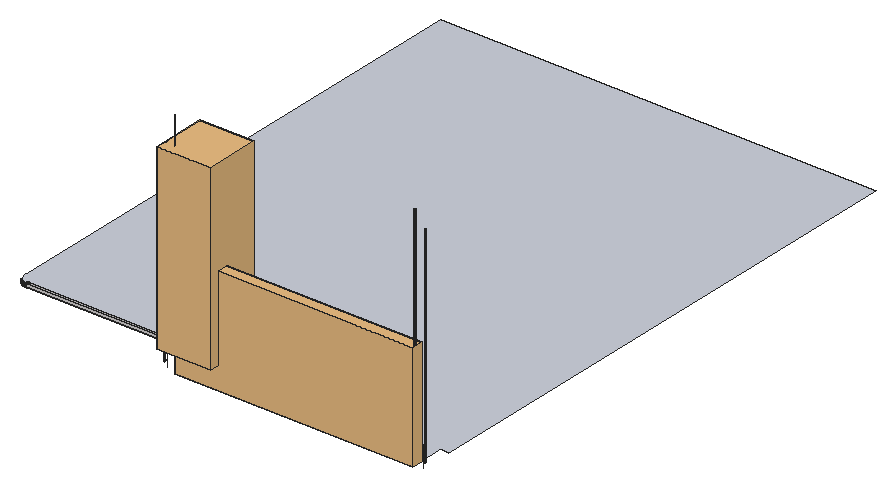
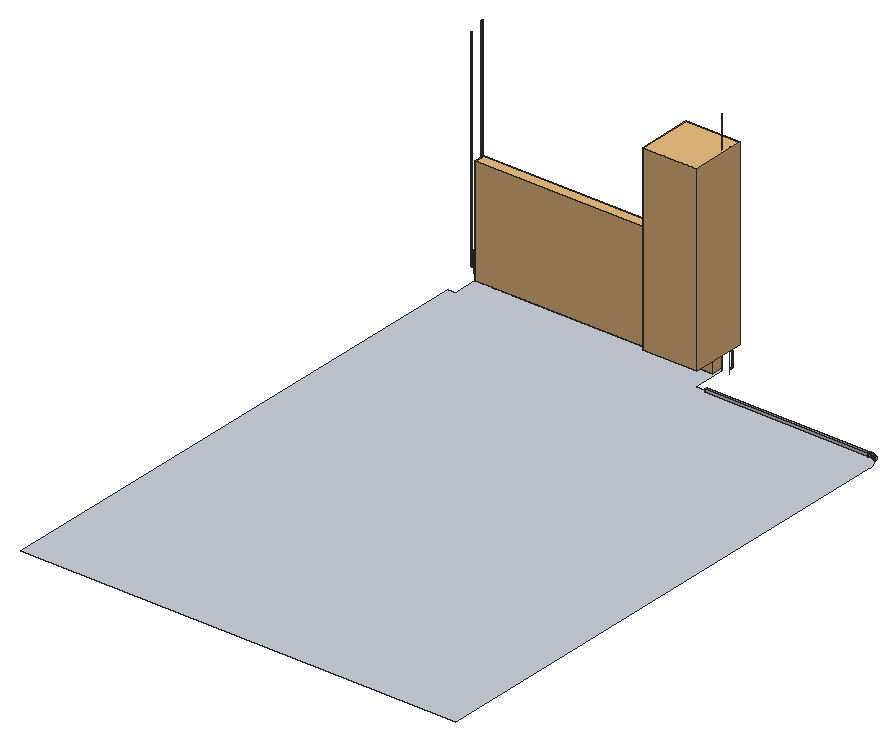
# SketchUp Ruby script. Lengths in inches.
U = 1.inch
M = Sketchup.active_model
def pt(a) = Geom::Point3d.new(a.map { |v| v * U })
def face(e, loops, mat)
  f = e.add_face(loops[0].map { |a| pt(a) })
  loops[1..].each { |l| e.add_face(l.map { |a| pt(a) }).erase! }
  f.material = f.back_material = mat if mat
  f
end
# faces: each face lists its corners as indices into pts; further lists are holes
def faces(e, pts, list, mat = nil) = list.each { |f| face(e, (f[0].is_a?(Array) ? f : [f]).map { |l| l.map { |i| pts[i] } }, mat) }
# xy, xz, yz: faces in a plane at the given z, y or x. An outline is a flat list of corners, or four numbers for a rectangle; further outlines are holes
def ring(l) = l.size == 4 ? [[l[0], l[1]], [l[2], l[1]], [l[2], l[3]], [l[0], l[3]]] : l.each_slice(2).to_a
def flat(e, list, mat, &to3) = list.each { |f| face(e, (f[0].is_a?(Array) ? f : [f]).map { |l| ring(l).map { |u, v| to3.(u, v) } }, mat) }
def xy(e, z, list, mat = nil) = flat(e, list, mat) { |x, y| [x, y, z] }
def xz(e, y, list, mat = nil) = flat(e, list, mat) { |x, z| [x, y, z] }
def yz(e, x, list, mat = nil) = flat(e, list, mat) { |y, z| [x, y, z] }
def lines(e, pts, list) = list.each { |a, b| e.add_line(pt(pts[a]), pt(pts[b])) }
# prism: a flat outline (further loops are holes) pulled along v
def prism(e, loops, v, mat = nil)
  f = face(e, loops, mat); d = Geom::Vector3d.new(v.map { |x| x * U })
  f.pushpull(f.normal.samedirection?(d) ? d.length : -d.length)
end
def box(e, o, s, mat = nil) = prism(e, [[o, [o[0] + s[0], o[1], o[2]], [o[0] + s[0], o[1] + s[1], o[2]], [o[0], o[1] + s[1], o[2]]]], [0, 0, s[2]], mat)
def at(x, y, z, deg = 0) = Geom::Transformation.translation(pt([x, y, z])) * Geom::Transformation.rotation(ORIGIN, Z_AXIS, deg.degrees)
def axes(o, x, y, z) = Geom::Transformation.new([*x, 0, *y, 0, *z, 0, *pt(o).to_a, 1])
def part(name) = M.definitions.add(name)
# library, detail: a bought-in or finely detailed component or shape, given as its bounding box
def library(name, o, s) = part(name).tap { |d| box(d.entities, o, s) }
def detail(e, o, s) = box(e.add_group.entities, o, s)
def put(e, d, t, mat = nil) = e.add_instance(d, t).tap { |i| i.material = mat if mat }
def group(e, t, mat = nil) = e.add_group.tap { |g| g.transformation = t; g.material = mat if mat }.entities
root = M.entities
M.materials.add("[Marble Carrara Floor Tile]").color = [204, 208, 219]
M.materials.add("[Quartz Light Brown]").color = [215, 212, 212]
M.materials.add("[Wood Cherry Original]").color = [152, 86, 42]
c1 = library("Garniza_zaclona",[1.52,0,0],[127.96,8.15,78.72])
c2 = library("Group\#4",[-1.08,-1,0],[60.58,61,204])
xy(root,126,[[216,155,480.079,155,480.192,155.005,480.306,155.015,480.419,155.028,480.531,155.046,480.643,155.069,480.754,155.095,480.863,155.126,480.972,155.161,481.079,155.2,481.184,155.243,481.288,155.29,481.39,155.341,481.49,155.395,481.588,155.454,481.683,155.516,481.776,155.582,481.867,155.651,481.955,155.723,482.04,155.799,482.122,155.878,482.201,155.96,482.276,156.045,482.349,156.133,482.418,156.224,482.484,156.317,482.546,156.412,482.604,156.51,482.659,156.61,482.71,156.712,482.757,156.815,482.8,156.921,482.838,157.028,482.873,157.136,482.904,157.246,482.93,157.357,482.953,157.469,482.971,157.581,482.984,157.694,482.994,157.808,482.999,157.921,483,194,492,194,492,794,3,794,3,212,3.001,211.804,3.005,211.607,3.012,211.411,3.021,211.215,3.032,211.019,3.046,210.823,3.063,210.627,3.082,210.432,3.104,210.237,3.128,210.042,3.155,209.848,3.185,209.653,3.217,209.46,3.251,209.266,3.288,209.074,3.328,208.881,3.37,208.69,3.414,208.498,3.462,208.308,3.511,208.118,3.563,207.928,3.618,207.74,3.675,207.552,3.734,207.365,3.796,207.178,3.86,206.993,3.927,206.808,3.996,206.624,4.068,206.442,4.142,206.26,4.218,206.079,4.297,205.899,4.378,205.72,4.461,205.542,4.547,205.366,4.635,205.19,4.725,205.016,4.818,204.843,4.913,204.671,5.01,204.5,5.109,204.331,5.21,204.163,5.314,203.996,5.42,203.83,5.528,203.666,5.638,203.504,5.75,203.343,5.865,203.183,5.981,203.025,6.1,202.869,6.22,202.714,6.343,202.56,6.467,202.408,6.594,202.258,6.722,202.11,6.853,201.963,6.985,201.818,7.119,201.675,7.255,201.533,7.393,201.393,7.533,201.255,7.675,201.119,7.818,200.985,7.963,200.853,8.11,200.722,8.258,200.594,8.408,200.467,8.56,200.343,8.714,200.22,8.869,200.1,9.025,199.981,9.183,199.865,9.343,199.75,9.504,199.638,9.666,199.528,9.83,199.42,9.996,199.314,10.163,199.21,10.331,199.109,10.5,199.01,10.671,198.913,10.843,198.818,11.016,198.725,11.19,198.635,11.366,198.547,11.542,198.461,11.72,198.378,11.899,198.297,12.079,198.218,12.26,198.142,12.442,198.068,12.624,197.996,12.808,197.927,12.993,197.86,13.178,197.796,13.365,197.734,13.552,197.675,13.74,197.618,13.928,197.563,14.118,197.511,14.308,197.462,14.498,197.414,14.69,197.37,14.881,197.328,15.074,197.288,15.266,197.251,15.46,197.217,15.653,197.185,15.848,197.155,16.042,197.128,16.237,197.104,16.432,197.082,16.627,197.063,16.823,197.046,17.019,197.032,17.215,197.021,17.411,197.012,17.607,197.005,17.804,197.001,18,197,201,197,201,194,213,194,213,158,213.002,157.882,213.009,157.765,213.021,157.647,213.037,157.531,213.058,157.415,213.083,157.3,213.113,157.186,213.147,157.073,213.186,156.962,213.229,156.852,213.276,156.744,213.327,156.638,213.383,156.534,213.442,156.433,213.506,156.333,213.573,156.237,213.644,156.143,213.719,156.052,213.797,155.964,213.879,155.879,213.964,155.797,214.052,155.719,214.143,155.644,214.237,155.573,214.333,155.506,214.433,155.442,214.534,155.383,214.638,155.327,214.744,155.276,214.852,155.228,214.962,155.185,215.073,155.147,215.186,155.113,215.3,155.083,215.415,155.058,215.531,155.037,215.648,155.021,215.765,155.009,215.882,155.002]],"[Marble Carrara Floor Tile]")
xz(root,194,[[18,126,201,129]],"[Quartz Light Brown]")
xz(root,194.5,[[18.002,125,201,126]],"[Quartz Light Brown]")
xz(root,197,[[18,126,201,129]],"[Quartz Light Brown]")
yz(root,201,[[194,125,194.5,126],[194,126,197,129]],"[Quartz Light Brown]")
yz(root,482.996,[[157.843,126,157.846,384]],"[Quartz Light Brown]")
p = [[16.627,194.554,126],[16.627,194.554,125],[16.855,194.537,125],[16.855,194.537,126],[17.084,194.524,125],[17.084,194.524,126],
  [17.313,194.514,125],[17.313,194.514,126],[17.542,194.506,125],[17.542,194.506,126],[17.771,194.502,125],[17.771,194.502,126],
  [18.002,194.5,125],[18.002,194.5,126],[15.489,194.681,126],[15.489,194.681,125],[15.716,194.65,125],[15.716,194.65,126],
  [15.943,194.621,125],[15.943,194.621,126],[16.171,194.596,125],[16.171,194.596,126],[16.399,194.573,125],[16.399,194.573,126],
  [15.036,194.753,126],[15.036,194.753,125],[15.262,194.715,125],[15.262,194.715,126],[14.362,194.882,126],[14.362,194.882,125],
  [14.586,194.836,125],[14.586,194.836,126],[14.811,194.793,125],[14.811,194.793,126],[13.915,194.984,126],[13.915,194.984,125],
  [14.138,194.932,125],[14.138,194.932,126],[13.471,195.096,126],[13.471,195.096,125],[13.692,195.038,125],[13.692,195.038,126],
  [13.25,195.157,126],[13.25,195.157,125],[12.811,195.287,126],[12.811,195.287,125],[13.03,195.221,125],[13.03,195.221,126],
  [12.592,195.357,126],[12.592,195.357,125],[12.158,195.504,126],[12.158,195.504,125],[12.375,195.429,125],[12.375,195.429,126],
  [11.943,195.582,126],[11.943,195.582,125],[11.729,195.662,126],[11.729,195.662,125],[11.303,195.832,126],[11.303,195.832,125],
  [11.515,195.746,125],[11.515,195.746,126],[11.092,195.921,126],[11.092,195.921,125],[10.882,196.013,126],[10.882,196.013,125],
  [10.673,196.108,126],[10.673,196.108,125],[10.466,196.205,126],[10.466,196.205,125],[10.26,196.305,126],[10.26,196.305,125],
  [10.055,196.407,126],[10.055,196.407,125],[9.852,196.513,126],[9.852,196.513,125],[9.65,196.621,126],[9.65,196.621,125],
  [9.449,196.731,126],[9.449,196.731,125],[9.25,196.845,126],[9.25,196.845,125],[9.052,196.96,126],[9.052,196.96,125],
  [8.856,197.079,126],[8.856,197.079,125],[8.662,197.2,126],[8.662,197.2,125],[8.469,197.323,126],[8.469,197.323,125],
  [8.278,197.449,126],[8.278,197.449,125],[213.506,156.333,384],[213.528,156.301,384],[213.528,156.301,126],[213.506,156.333,126],
  [213.484,156.366,384],[213.484,156.366,126],[482.494,156.333,384],[482.498,156.338,384],[482.498,156.338,126],[482.494,156.333,126],
  [482.516,156.366,126],[482.516,156.366,384],[213.442,156.433,384],[213.463,156.399,384],[213.463,156.399,126],[213.442,156.433,126],
  [213.422,156.466,384],[213.422,156.466,126],[482.537,156.399,384],[482.537,156.399,126],[482.541,156.405,384],[482.558,156.433,384],
  [482.558,156.433,126],[482.56,156.435,384],[482.56,156.435,126],[482.578,156.466,126],[482.576,156.462,384],[482.578,156.466,384],
  [213.402,156.5,384],[213.402,156.5,126],[213.383,156.534,384],[213.383,156.534,126],[213.364,156.569,384],[213.364,156.569,126],
  [482.598,156.5,384],[482.598,156.5,126],[482.602,156.507,384],[482.617,156.534,384],[482.617,156.534,126],[482.632,156.561,384],
  [482.636,156.569,384],[482.636,156.569,126],[213.345,156.603,384],[213.345,156.603,126],[213.327,156.638,384],[213.327,156.638,126],
  [213.309,156.673,384],[213.309,156.673,126],[482.655,156.603,384],[482.655,156.603,126],[482.659,156.61,384],[482.672,156.635,384],
  [482.672,156.635,126],[482.673,156.638,126],[482.673,156.638,384],[482.684,156.661,384],[482.691,156.673,384],[482.691,156.673,126],
  [213.292,156.708,384],[213.292,156.708,126],[213.276,156.744,384],[213.276,156.744,126],[213.259,156.78,384],[213.259,156.78,126],
  [482.708,156.708,384],[482.708,156.708,126],[482.711,156.716,384],[482.722,156.738,384],[482.722,156.738,126],[482.724,156.744,126],
  [482.724,156.744,384],[482.732,156.762,384],[482.741,156.78,384],[482.741,156.78,126],[213.244,156.816,384],[213.244,156.816,126],
  [213.228,156.852,384],[213.228,156.852,126],[482.756,156.816,384],[482.756,156.816,126],[482.76,156.823,384],[482.768,156.843,384],
  [482.768,156.843,126],[482.772,156.852,126],[482.772,156.852,384],[213.214,156.888,384],[213.214,156.888,126],[213.199,156.925,384],
  [213.199,156.925,126],[213.185,156.962,384],[213.185,156.962,126],[482.777,156.864,384],[482.786,156.888,384],[482.786,156.888,126],
  [482.801,156.925,384],[482.801,156.925,126],[482.804,156.932,384],[482.811,156.95,384],[482.81,156.95,126],[213.147,157.073,384],
  [213.159,157.036,384],[213.159,157.036,126],[213.147,157.073,126],[213.172,156.999,384],[213.172,156.999,126],[482.815,156.962,126],
  [482.815,156.962,384],[482.816,156.967,384],[482.828,156.999,384],[482.828,156.999,126],[482.841,157.036,384],[482.841,157.036,126],
  [482.843,157.043,384],[482.849,157.058,384],[482.849,157.058,126],[213.135,157.11,384],[213.135,157.11,126],[213.124,157.148,384],
  [213.124,157.148,126],[213.113,157.186,384],[213.113,157.186,126],[482.853,157.073,126],[482.853,157.071,384],[482.853,157.073,384],
  [482.865,157.11,384],[482.865,157.11,126],[482.876,157.148,384],[482.876,157.148,126],[482.878,157.155,384],[482.883,157.168,384],
  [482.882,157.168,126],[213.102,157.224,384],[213.102,157.224,126],[213.092,157.262,384],[213.092,157.262,126],[482.887,157.186,126],
  [482.886,157.18,384],[482.887,157.186,384],[482.898,157.224,384],[482.898,157.224,126],[482.908,157.262,384],[482.908,157.262,126],
  [213.083,157.3,384],[213.083,157.3,126],[213.074,157.338,384],[213.074,157.338,126],[213.066,157.376,384],[213.066,157.376,126],
  [482.909,157.268,384],[482.912,157.279,384],[482.912,157.279,126],[482.917,157.3,126],[482.915,157.29,384],[482.917,157.3,384],
  [482.926,157.338,384],[482.926,157.338,126],[482.934,157.376,384],[482.934,157.376,126],[213.058,157.415,384],[213.058,157.415,126],
  [213.05,157.453,384],[213.05,157.453,126],[482.936,157.382,384],[482.9375,157.391,384],[482.9375,157.391,126],[482.942,157.415,126],
  [482.94,157.401,384],[482.942,157.415,384],[482.95,157.453,384],[482.95,157.453,126],[213.043,157.492,384],[213.043,157.492,126],
  [213.037,157.531,384],[213.037,157.531,126],[213.031,157.57,384],[213.031,157.57,126],[482.957,157.492,384],[482.957,157.492,126],
  [482.958,157.497,384],[482.959,157.504,384],[482.959,157.504,126],[482.963,157.531,126],[482.96,157.512,384],[482.963,157.531,384],
  [482.969,157.57,384],[482.969,157.57,126],[213.026,157.608,384],[213.026,157.608,126],[213.021,157.647,384],[213.021,157.647,126],
  [213.016,157.686,384],[213.016,157.686,126],[482.974,157.608,384],[482.974,157.608,126],[482.975,157.613,384],[482.976,157.617,384],
  [482.976,157.617,126],[482.979,157.647,126],[482.976,157.623,384],[482.979,157.647,384],[482.984,157.686,384],[482.984,157.686,126],
  [213.013,157.725,384],[213.013,157.725,126],[213.009,157.765,384],[213.009,157.765,126],[482.987,157.725,384],[482.987,157.725,126],
  [482.988,157.729,384],[482.988,157.731,384],[482.988,157.731,126],[482.991,157.765,126],[482.988,157.735,384],[482.991,157.765,384],
  [213.006,157.804,384],[213.006,157.804,126],[213.004,157.843,384],[213.004,157.843,126],[213.002,157.881,126],[213.003,157.881,384],
  [482.994,157.804,384],[482.994,157.804,126],[482.996,157.843,384],[482.996,157.843,126],[482.998,157.882,126],[482.996,157.846,126],
  [482.996,157.846,384],[482.998,157.882,384],[213.002,157.882,384],[213.002,157.882,126],[213.001,157.921,384],[213.001,157.921,126],
  [482.999,157.921,384],[482.999,157.921,126],[16.823,194.039,126],[16.823,194.039,129],[16.588,194.055,129],[16.588,194.055,126],
  [17.058,194.025,126],[17.058,194.025,129],[17.293,194.014,126],[17.293,194.014,129],[17.529,194.006,126],[17.529,194.006,129],
  [17.764,194.002,126],[17.764,194.002,129],[18,194,126],[18,194,129],[15.884,194.125,126],[15.884,194.125,129],
  [15.651,194.154,129],[15.651,194.154,126],[16.118,194.099,126],[16.118,194.099,129],[16.353,194.076,126],[16.353,194.076,129],
  [15.184,194.222,126],[15.184,194.222,129],[14.952,194.26,129],[14.952,194.26,126],[15.417,194.186,126],[15.417,194.186,129],
  [14.488,194.346,126],[14.488,194.346,129],[14.258,194.393,129],[14.258,194.393,126],[14.72,194.301,126],[14.72,194.301,129],
  [14.027,194.444,126],[14.027,194.444,129],[13.798,194.497,129],[13.798,194.497,126],[13.569,194.554,129],[13.569,194.554,126],
  [13.341,194.613,126],[13.341,194.613,129],[13.114,194.676,129],[13.114,194.676,126],[12.888,194.741,126],[12.888,194.741,129],
  [12.662,194.81,129],[12.662,194.81,126],[12.4375,194.881,129],[12.4375,194.881,126],[12.214,194.955,129],[12.214,194.955,126],
  [11.991,195.032,126],[11.991,195.032,129],[11.77,195.113,129],[11.77,195.113,126],[11.549,195.196,129],[11.549,195.196,126],
  [11.33,195.281,129],[11.33,195.281,126],[11.112,195.37,129],[11.112,195.37,126],[10.895,195.462,129],[10.895,195.462,126],
  [10.679,195.556,129],[10.679,195.556,126],[10.464,195.653,129],[10.464,195.653,126],[10.251,195.753,129],[10.251,195.753,126],
  [10.039,195.856,129],[10.039,195.856,126],[9.828,195.962,129],[9.828,195.962,126],[9.619,196.07,129],[9.619,196.07,126],
  [9.411,196.181,129],[9.411,196.181,126],[9.205,196.295,129],[9.205,196.295,126],[9,196.412,129],[9,196.412,126],
  [8.797,196.531,129],[8.797,196.531,126],[8.595,196.652,129],[8.595,196.652,126],[8.395,196.777,129],[8.395,196.777,126],
  [8.196,196.904,129],[8.196,196.904,126],[8,197.034,129],[8,197.034,126],[7.805,197.166,129],[7.805,197.166,126],
  [16.823,197.046,126],[16.627,197.063,126],[16.627,197.063,129],[16.823,197.046,129],[17.019,197.032,126],[17.019,197.032,129],
  [17.215,197.021,126],[17.215,197.021,129],[17.411,197.012,126],[17.411,197.012,129],[17.607,197.005,126],[17.607,197.005,129],
  [17.804,197.001,126],[17.804,197.001,129],[18,197,126],[18,197,129],[16.042,197.128,126],[15.848,197.155,126],
  [15.848,197.155,129],[16.042,197.128,129],[16.237,197.104,126],[16.237,197.104,129],[16.432,197.082,126],[16.432,197.082,129],
  [7.611,197.3,129],[7.611,197.3,126],[15.46,197.217,126],[15.266,197.251,126],[15.266,197.251,129],[15.46,197.217,129],
  [15.653,197.185,126],[15.653,197.185,129],[7.42,197.4375,129],[7.42,197.4375,126],[14.881,197.328,126],[14.69,197.37,126],
  [14.69,197.37,129],[14.881,197.328,129],[15.074,197.288,126],[15.074,197.288,129],[202.077,156.537,133],[202.077,156.537,132],
  [202.097,156.354,132],[202.097,156.354,133],[493.903,156.354,133],[493.903,156.354,132],[493.923,156.537,132],[493.923,156.537,133],
  [202.059,156.719,133],[202.059,156.719,132],[493.941,156.719,132],[493.941,156.719,133],[202.043,156.902,133],[202.043,156.902,132],
  [493.957,156.902,132],[493.957,156.902,133],[202.03,157.084,133],[202.03,157.084,132],[493.97,157.084,132],[493.97,157.084,133],
  [202.019,157.267,133],[202.019,157.267,132],[493.981,157.267,132],[493.981,157.267,133],[202.011,157.45,133],[202.011,157.45,132],
  [493.989,157.45,132],[493.989,157.45,133],[202.005,157.634,133],[202.005,157.634,132],[493.995,157.634,132],[493.995,157.634,133],
  [202.001,157.817,133],[202.001,157.817,132],[493.999,157.817,132],[493.999,157.817,133],[202,158.003,133],[202,158.003,132],
  [494,158.003,132],[494,158.003,133],[201.104,156.237,133],[201.104,156.237,150],[201.082,156.432,150],[201.082,156.432,133],
  [494.896,156.237,368],[494.896,156.237,133],[494.918,156.432,133],[494.918,156.432,368],[201.063,156.627,150],[201.063,156.627,133],
  [494.937,156.627,133],[494.937,156.627,368],[201.046,156.823,150],[201.046,156.823,133],[494.954,156.823,133],[494.954,156.823,368],
  [201.032,157.019,150],[201.032,157.019,133],[494.968,157.019,133],[494.968,157.019,368],[201.021,157.215,150],[201.021,157.215,133],
  [494.979,157.215,133],[494.979,157.215,368],[201.012,157.411,150],[201.012,157.411,133],[494.988,157.411,133],[494.988,157.411,368],
  [201.005,157.607,150],[201.005,157.607,133],[494.995,157.607,133],[494.995,157.607,368],[201.001,157.804,150],[201.001,157.804,133],
  [494.999,157.804,133],[494.999,157.804,368],[201,158,150],[201,158,133],[495,158,133],[495,158,368],
  [201.828,156.51,150],[201.849,156.325,150],[201.849,156.325,149.75],[201.828,156.51,149.75],[202.345,156.384,150],[202.325,156.563,150],
  [202.325,156.563,149.75],[202.345,156.384,149.75],[201.81,156.696,150],[201.81,156.696,149.75],[202.308,156.742,150],[202.308,156.742,149.75],
  [201.794,156.882,150],[201.794,156.882,149.75],[202.292,156.921,150],[202.292,156.921,149.75],[201.781,157.068,150],[201.781,157.068,149.75],
  [202.279,157.101,150],[202.279,157.101,149.75],[201.77,157.254,150],[201.77,157.254,149.75],[202.269,157.28,150],[202.269,157.28,149.75],
  [201.761,157.441,150],[201.761,157.441,149.75],[202.261,157.46,150],[202.261,157.46,149.75],[201.755,157.627,150],[201.755,157.627,149.75],
  [202.255,157.64,150],[202.255,157.64,149.75],[201.751,157.813,150],[201.751,157.813,149.75],[202.251,157.82,150],[202.251,157.82,149.75],
  [201.75,158,150],[201.75,158,149.75],[202.25,158,150],[202.25,158,149.75],[204.124,156.278,150],[204.124,156.278,354],
  [204.103,156.434,354],[204.103,156.434,150],[204.083,156.59,354],[204.083,156.59,150],[204.066,156.746,354],[204.066,156.746,150],
  [204.05,156.902,354],[204.05,156.902,150],[204.037,157.058,354],[204.037,157.058,150],[204.026,157.215,354],[204.026,157.215,150],
  [204.016,157.372,354],[204.016,157.372,150],[204.009,157.529,354],[204.009,157.529,150],[204.004,157.686,354],[204.004,157.686,150],
  [204.001,157.843,354],[204.001,157.843,150],[204,158,354],[204,158,150],[492,158,150],[492,158,126],
  [204,158,126],[491.876,156.278,150],[491.897,156.434,150],[491.917,156.59,150],[491.934,156.746,150],[491.95,156.902,150],
  [491.963,157.058,150],[491.974,157.215,150],[491.984,157.372,150],[491.991,157.529,150],[491.996,157.686,150],[491.999,157.843,150]]
faces(root,p,[[0,1,2,3],[3,2,4,5],[5,4,6,7],[7,6,8,9],[9,8,10,11],[11,10,12,13],[14,15,16,17],[17,16,18,19],
  [19,18,20,21],[21,20,22,23],[23,22,1,0],[24,25,26,27],[27,26,15,14],[28,29,30,31],[31,30,32,33],[33,32,25,24],
  [34,35,36,37],[37,36,29,28],[38,39,40,41],[41,40,35,34],[42,43,39,38],[44,45,46,47],[47,46,43,42],[48,49,45,44],
  [50,51,52,53],[53,52,49,48],[54,55,51,50],[56,57,55,54],[58,59,60,61],[61,60,57,56],[62,63,59,58],[64,65,63,62],
  [66,67,65,64],[68,69,67,66],[70,71,69,68],[72,73,71,70],[74,75,73,72],[76,77,75,74],[78,79,77,76],[80,81,79,78],
  [82,83,81,80],[84,85,83,82],[86,87,85,84],[88,89,87,86],[90,91,89,88],[92,93,94,95],[96,92,95,97],[98,99,100,101],
  [102,100,99,103],[104,105,106,107],[108,104,107,109],[105,96,97,106],[103,110,111,102],[110,112,113,114,111],[113,115,116,114],[117,116,115,118,119],
  [120,108,109,121],[122,120,121,123],[124,122,123,125],[119,126,127,117],[126,128,129,130,127],[129,131,132,133,130],[134,124,125,135],[136,134,135,137],
  [138,136,137,139],[132,140,141,133],[142,143,144,141,140],[145,144,143,146],[146,147,148,149,145],[150,138,139,151],[152,150,151,153],[154,152,153,155],
  [148,156,157,149],[158,159,160,157,156],[161,160,159,162],[162,163,164,165,161],[166,154,155,167],[168,166,167,169],[164,170,171,165],[172,173,174,171,170],
  [175,174,173,176],[177,168,169,178],[179,177,178,180],[181,179,180,182],[176,183,184,185,175],[184,186,187,185],[188,189,190,187,186],[191,192,193,194],
  [195,181,182,196],[195,192,193,196],[197,190,189,198],[198,199,200,201,197],[200,202,203,201],[204,205,206,203,202],[207,191,194,208],[207,209,210,208],
  [211,209,210,212],[213,206,205,214,215],[215,216,217,213],[216,218,219,217],[220,221,222,219,218],[223,211,212,224],[225,223,224,226],[227,222,221,228,229],
  [229,230,231,227],[230,232,233,231],[234,225,226,235],[236,234,235,237],[238,236,237,239],[240,241,242,233,232],[243,242,241,244,245],[245,246,247,243],
  [246,248,249,247],[250,238,239,251],[252,250,251,253],[254,255,256,249,248],[257,256,255,258,259],[259,260,261,257],[262,252,253,263],[264,262,263,265],
  [266,264,265,267],[260,268,269,261],[270,271,272,269,268],[273,272,271,274,275],[275,276,277,273],[278,266,267,279],[280,278,279,281],[282,280,281,283],
  [276,284,285,277],[286,287,288,285,284],[289,288,287,290,291],[291,292,293,289],[294,282,283,295],[296,294,295,297],[292,298,299,293],[300,301,302,299,298],
  [303,302,301,304,305],[306,296,297,307],[308,306,307,309],[309,310,311,308],[305,312,313,303],[312,314,315,313],[316,317,318,319],[320,311,310,321],
  [322,320,321,323],[319,324,325,316],[326,327,328,329],[330,331,327,326],[332,333,331,330],[334,335,333,332],[336,337,335,334],[338,339,337,336],
  [340,341,342,343],[344,345,341,340],[346,347,345,344],[329,328,347,346],[348,349,350,351],[352,353,349,348],[343,342,353,352],[354,355,356,357],
  [358,359,355,354],[351,350,359,358],[360,361,362,363],[357,356,361,360],[363,362,364,365],[366,367,368,369],[365,364,367,366],[370,371,372,373],
  [369,368,371,370],[373,372,374,375],[375,374,376,377],[378,379,380,381],[377,376,379,378],[381,380,382,383],[383,382,384,385],[385,384,386,387],
  [387,386,388,389],[389,388,390,391],[391,390,392,393],[393,392,394,395],[395,394,396,397],[397,396,398,399],[399,398,400,401],[401,400,402,403],
  [403,402,404,405],[405,404,406,407],[407,406,408,409],[409,408,410,411],[411,410,412,413],[413,412,414,415],[415,414,416,417],[417,416,418,419],
  [420,421,422,423],[424,420,423,425],[426,424,425,427],[428,426,427,429],[430,428,429,431],[432,430,431,433],[434,432,433,435],[436,437,438,439],
  [440,436,439,441],[442,440,441,443],[421,442,443,422],[419,418,444,445],[446,447,448,449],[450,446,449,451],[437,450,451,438],[445,444,452,453],
  [454,455,456,457],[458,454,457,459],[447,458,459,448],[460,461,462,463],[464,465,466,467],[468,469,461,460],[467,466,470,471],[472,473,469,468],
  [471,470,474,475],[476,477,473,472],[475,474,478,479],[480,481,477,476],[479,478,482,483],[484,485,481,480],[483,482,486,487],[488,489,485,484],
  [487,486,490,491],[492,493,489,488],[491,490,494,495],[496,497,493,492],[495,494,498,499],[500,501,502,503],[504,505,506,507],[503,502,508,509],
  [507,506,510,511],[509,508,512,513],[511,510,514,515],[513,512,516,517],[515,514,518,519],[517,516,520,521],[519,518,522,523],[521,520,524,525],
  [523,522,526,527],[525,524,528,529],[527,526,530,531],[529,528,532,533],[531,530,534,535],[533,532,536,537],[535,534,538,539],[540,541,542,543],
  [544,545,546,547],[548,540,543,549],[545,550,551,546],[552,548,549,553],[550,554,555,551],[556,552,553,557],[554,558,559,555],[560,556,557,561],
  [558,562,563,559],[564,560,561,565],[562,566,567,563],[568,564,565,569],[566,570,571,567],[572,568,569,573],[570,574,575,571],[576,572,573,577],
  [574,578,579,575],[580,581,582,583],[583,582,584,585],[585,584,586,587],[587,586,588,589],[589,588,590,591],[591,590,592,593],[593,592,594,595],
  [595,594,596,597],[597,596,598,599],[599,598,600,601],[601,600,602,603]],"[Quartz Light Brown]")
lines(root,p,[[604,605],[603,606],[607,608],[608,609],[609,610],[610,611],[611,612],[612,613],[613,614],[614,615],[615,616],[616,617],
  [617,604]])
put(root,c1,axes([213,154.04,126],[2.08532,0,0],[0,1.49,0],[0,0,1.52445]))
put(root,c2,axes([204,145.6,150],[1,0,0],[0,0.99,0],[0,0,1]),"[Wood Cherry Original]")
